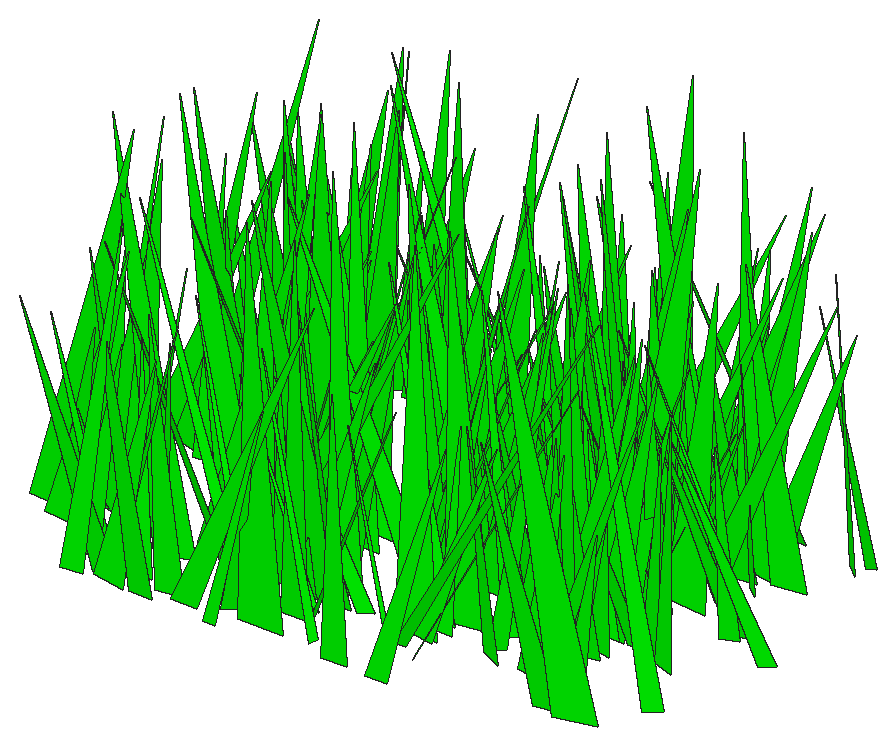
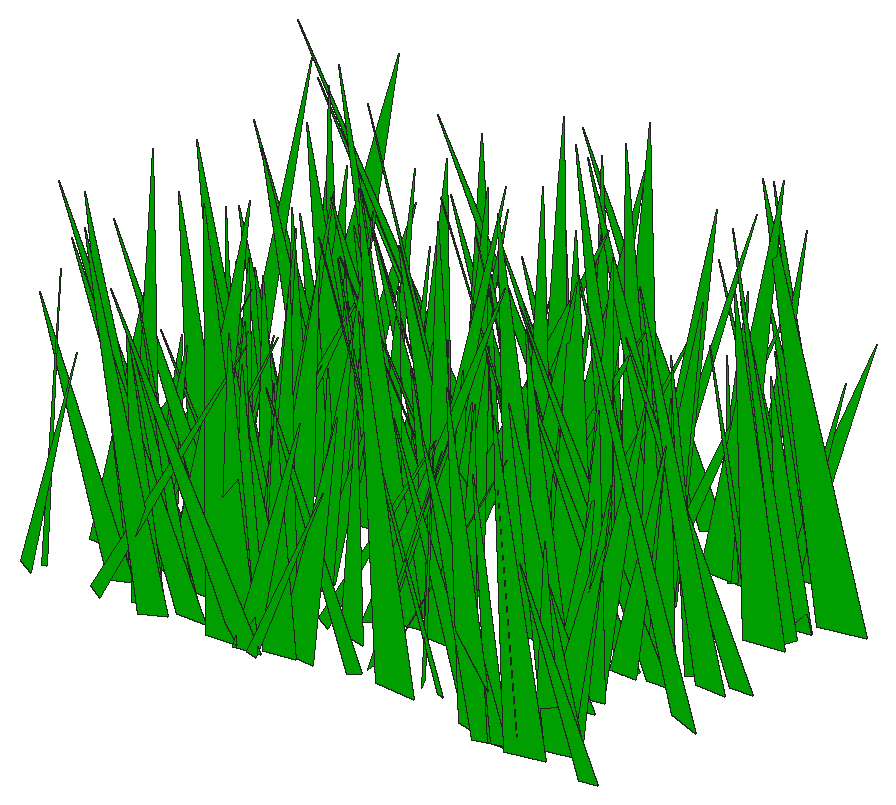
# SketchUp Ruby script. Lengths in inches.
U = 1.inch
M = Sketchup.active_model
def pt(a) = Geom::Point3d.new(a.map { |v| v * U })
def face(e, loops, mat)
  f = e.add_face(loops[0].map { |a| pt(a) })
  loops[1..].each { |l| e.add_face(l.map { |a| pt(a) }).erase! }
  f.material = f.back_material = mat if mat
  f
end
# faces: each face lists its corners as indices into pts; further lists are holes
def faces(e, pts, list, mat = nil) = list.each { |f| face(e, (f[0].is_a?(Array) ? f : [f]).map { |l| l.map { |i| pts[i] } }, mat) }
# xy, xz, yz: faces in a plane at the given z, y or x. An outline is a flat list of corners, or four numbers for a rectangle; further outlines are holes
def ring(l) = l.size == 4 ? [[l[0], l[1]], [l[2], l[1]], [l[2], l[3]], [l[0], l[3]]] : l.each_slice(2).to_a
def flat(e, list, mat, &to3) = list.each { |f| face(e, (f[0].is_a?(Array) ? f : [f]).map { |l| ring(l).map { |u, v| to3.(u, v) } }, mat) }
def xy(e, z, list, mat = nil) = flat(e, list, mat) { |x, y| [x, y, z] }
def xz(e, y, list, mat = nil) = flat(e, list, mat) { |x, z| [x, y, z] }
def yz(e, x, list, mat = nil) = flat(e, list, mat) { |y, z| [x, y, z] }
def lines(e, pts, list) = list.each { |a, b| e.add_line(pt(pts[a]), pt(pts[b])) }
# prism: a flat outline (further loops are holes) pulled along v
def prism(e, loops, v, mat = nil)
  f = face(e, loops, mat); d = Geom::Vector3d.new(v.map { |x| x * U })
  f.pushpull(f.normal.samedirection?(d) ? d.length : -d.length)
end
def box(e, o, s, mat = nil) = prism(e, [[o, [o[0] + s[0], o[1], o[2]], [o[0] + s[0], o[1] + s[1], o[2]], [o[0], o[1] + s[1], o[2]]]], [0, 0, s[2]], mat)
def at(x, y, z, deg = 0) = Geom::Transformation.translation(pt([x, y, z])) * Geom::Transformation.rotation(ORIGIN, Z_AXIS, deg.degrees)
def axes(o, x, y, z) = Geom::Transformation.new([*x, 0, *y, 0, *z, 0, *pt(o).to_a, 1])
def part(name) = M.definitions.add(name)
# library, detail: a bought-in or finely detailed component or shape, given as its bounding box
def library(name, o, s) = part(name).tap { |d| box(d.entities, o, s) }
def detail(e, o, s) = box(e.add_group.entities, o, s)
def put(e, d, t, mat = nil) = e.add_instance(d, t).tap { |i| i.material = mat if mat }
def group(e, t, mat = nil) = e.add_group.tap { |g| g.transformation = t; g.material = mat if mat }.entities
root = M.entities
M.materials.add("[0065_Lime]").color = [0, 255, 0]
c1 = part("fur_instance\#9")
p = [[0.8125,0,1.79],[0.67,-0.02,1.48],[0,-0.11,0],[0,0.11,0]]
faces(c1.entities,p,[[0,1,2,3]])
put(root,c1,axes([50.91,22.23,1.48],[-0.76695,0.80867,0.33759],[-5.73856,-0.11303,0.44668],[0.6003,-0.04733,4.70135]),"[0065_Lime]")
put(root,c1,axes([49.92,33.26,1.48],[2.52942,0.48808,0.58412],[-3.5394,0.33926,0.64151],[0.23083,-0.14633,3.43573]),"[0065_Lime]")
put(root,c1,axes([50.48,21.11,1.48],[-0.67256,-0.6845,0.19925],[4.74683,-0.09985,-0.89267],[1.12113,0.01212,3.89906]),"[0065_Lime]")
put(root,c1,axes([51.94,31.51,1.48],[-4.54403,0.38433,1.74925],[-3.22618,-0.65155,-0.74814],[1.30275,-0.27296,4.24871]),"[0065_Lime]")
put(root,c1,axes([49.74,21.47,1.48],[3.99395,-1.12369,1.36705],[8.17134,0.54771,-0.70957],[0.04674,0.26599,7.23614]),"[0065_Lime]")
put(root,c1,axes([52.3125,31.72,1.48],[-0.7268,-0.77449,0.53828],[5.51485,-0.09001,0.58705],[-0.63479,0.10476,4.48382]),"[0065_Lime]")
put(root,c1,axes([50.54,22.92,1.48],[7.98989,-0.14628,2.13973],[1.33822,1.17114,-0.62341],[-2.49252,0.15988,6.52429]),"[0065_Lime]")
put(root,c1,axes([51.04,23.54,1.48],[2.25533,-0.90203,2.17945],[6.94499,0.31435,-0.39545],[-0.3929,0.37864,5.52033]),"[0065_Lime]")
put(root,c1,axes([49.92,28.72,1.48],[7.6841,0.72682,1.04641],[-5.11442,1.09474,-0.63071],[-1.50059,-0.00934,7.50804]),"[0065_Lime]")
put(root,c1,axes([52.6875,20.2,1.48],[-4.48222,0.17938,1.02633],[-1.535,-0.63027,-0.74423],[0.93025,-0.17572,3.7171]),"[0065_Lime]")
put(root,c1,axes([50.85,22.25,1.48],[2.00716,0.68192,1.98592],[-5.43179,0.24636,0.79769],[0.08265,-0.36953,4.19657]),"[0065_Lime]")
put(root,c1,axes([50.48,20.87,1.48],[3.32906,-0.72326,1.49084],[5.46334,0.44405,-0.85316],[-0.06147,0.29661,4.91258]),"[0065_Lime]")
put(root,c1,axes([50.57,26.65,1.48],[-4.60892,-0.71981,3.549],[5.71561,-0.81095,-0.60041],[3.55095,0.37104,5.5728]),"[0065_Lime]")
put(root,c1,axes([51.49,26.26,1.48],[5.77813,-0.30698,2.05996],[2.54281,0.86465,-0.40144],[-2.17263,0.19556,5.00866]),"[0065_Lime]")
put(root,c1,axes([49.8125,26.12,1.48],[5.45246,0.6124,0.65614],[-4.43057,0.75796,0.65483],[-0.11992,-0.15925,5.63989]),"[0065_Lime]")
put(root,c1,axes([53.56,19.07,1.48],[-3.18516,-0.61642,0.82975],[4.4943,-0.42359,0.87005],[-0.29317,0.20357,4.32299]),"[0065_Lime]")
put(root,c1,axes([52.24,32.25,1.48],[-2.10277,0.6076,0.36206],[-4.26965,-0.30174,0.56101],[0.81554,-0.0131,3.87059]),"[0065_Lime]")
put(root,c1,axes([53.19,26.32,1.48],[-3.37771,-0.97874,1.73276],[7.26758,-0.4748,0.3867],[0.48409,0.29906,6.28475]),"[0065_Lime]")
put(root,c1,axes([53.32,28.98,1.48],[-3.44233,-0.75988,1.52882],[5.71042,-0.47776,0.55002],[0.40921,0.27472,5.18522]),"[0065_Lime]")
put(root,c1,axes([53.21,27.49,1.48],[-3.45068,0.52695,1.19509],[-3.97947,-0.48797,-0.39258],[0.62075,-0.19903,4.12659]),"[0065_Lime]")
put(root,c1,axes([52.51,26.5625,1.48],[-2.79875,-0.72297,0.6651],[5.04299,-0.4087,-0.84615],[1.30717,0.0288,4.68844]),"[0065_Lime]")
put(root,c1,axes([53.12,29.34,1.48],[-3.22496,0.8525,0.55277],[-6.03576,-0.46145,0.54834],[0.91558,-0.03923,5.56179]),"[0065_Lime]")
put(root,c1,axes([51.48,32.38,1.48],[1.93276,-0.94577,0.96552],[6.81569,0.25388,-0.69382],[0.50636,0.19268,5.6536]),"[0065_Lime]")
put(root,c1,axes([52.375,33.1875,1.48],[-1.67785,0.95461,1.59203],[-6.95575,-0.27347,0.64432],[1.2648,-0.23757,5.65537]),"[0065_Lime]")
put(root,c1,axes([53.34,30.1,1.48],[0.33738,-0.67966,0.71284],[4.87263,0.06252,0.47168],[-0.64838,0.1162,3.91559]),"[0065_Lime]")
put(root,c1,axes([52.05,22.86,1.48],[5.4099,-0.08173,1.18749],[0.45868,0.78549,0.42894],[-1.50305,-0.05446,4.40501]),"[0065_Lime]")
put(root,c1,axes([52.31,19.69,1.48],[-1.28397,0.58808,1.45449],[-4.36145,-0.23358,0.61725],[1.30018,-0.20279,3.50693]),"[0065_Lime]")
put(root,c1,axes([54.54,21.14,1.48],[-6.11177,0.83379,2.4404],[-6.48605,-0.87364,-0.74549],[1.46324,-0.38992,6.88873]),"[0065_Lime]")
put(root,c1,axes([52.62,18.63,1.48],[-6.04866,0.41876,3.20472],[-3.14623,-1.00131,0.45529],[3.80849,-0.16212,5.46587]),"[0065_Lime]")
put(root,c1,axes([52.71,29.97,1.48],[1.05104,0.56648,0.01025],[-3.99325,0.14604,0.46794],[0.55353,-0.02209,3.35635]),"[0065_Lime]")
put(root,c1,axes([53.35,32.34,1.48],[7.25224,0.0929,2.18108],[-0.93336,1.0789,0.51345],[-2.5992,-0.12821,5.90123]),"[0065_Lime]")
put(root,c1,axes([53.41,33.16,1.48],[4.50904,-0.4217,1.00213],[2.93431,0.65657,0.52272],[-1.38352,0.01815,4.37469]),"[0065_Lime]")
put(root,c1,axes([55.33,23.34,1.48],[-5.78731,0.88598,2.08157],[-6.6877,-0.82771,-0.49719],[1.25603,-0.32486,6.94378]),"[0065_Lime]")
put(root,c1,axes([55.17,18.71,1.48],[-5.21317,-0.59207,1.74612],[4.53951,-0.75234,0.41909],[1.32453,0.24817,5.4362]),"[0065_Lime]")
put(root,c1,axes([56.38,21.37,1.48],[-6.25595,-0.43733,0.00178],[3.07458,-0.86853,-0.87844],[0.48295,-0.13573,5.61532]),"[0065_Lime]")
put(root,c1,axes([54.44,19.73,1.48],[-3.81203,0.42571,0.97367],[-2.86432,-0.56136,0.80465],[1.55137,0.00959,3.87813]),"[0065_Lime]")
put(root,c1,axes([54.12,21.14,1.48],[-3.81363,-0.33001,1.35293],[2.07947,-0.58422,-0.89694],[1.98947,-0.02196,3.53096]),"[0065_Lime]")
put(root,c1,axes([52.01,27.33,1.48],[5.88229,0.64403,0.51482],[-4.62387,0.81322,0.86661],[0.16303,-0.17262,6.00343]),"[0065_Lime]")
put(root,c1,axes([54.34,33,1.48],[3.98604,0.93129,0.86549],[-6.54901,0.5777,-0.87367],[-1.47219,-0.04836,6.2299]),"[0065_Lime]")
put(root,c1,axes([53.92,18.77,1.48],[-0.50373,0.66106,1.56053],[-4.9413,-0.12675,0.74384],[1.18158,-0.24823,3.77598]),"[0065_Lime]")
put(root,c1,axes([55.15,26.55,1.48],[5.34275,-0.76963,2.59064],[5.69177,0.84019,0.5974],[-2.78312,0.24082,6.19498]),"[0065_Lime]")
put(root,c1,axes([55.07,26.01,1.48],[5.34106,0.58498,2.14604],[-4.12838,0.82961,-0.77951],[-2.6922,-0.11163,5.45286]),"[0065_Lime]")
put(root,c1,axes([53.03,27.32,1.48],[5.09999,-0.34369,0.51708],[2.52545,0.70055,-0.87733],[-0.09331,0.17544,4.51639]),"[0065_Lime]")
put(root,c1,axes([53.69,33.22,1.48],[2.05029,-0.79208,0.95149],[5.72232,0.26129,-0.86987],[0.63048,0.20433,4.8008]),"[0065_Lime]")
put(root,c1,axes([53.94,18.95,1.48],[5.8276,-0.01282,1.10697],[0.25412,0.83464,-0.56111],[-1.34008,0.1025,4.70751]),"[0065_Lime]")
put(root,c1,axes([54.94,23.94,1.48],[3.34017,-0.6062,0.80133],[4.24397,0.48796,0.66477],[-1.25297,0.03678,4.38788]),"[0065_Lime]")
put(root,c1,axes([55.77,19.33,1.48],[1.91514,0.72289,1.34833],[-5.21429,0.31216,-0.70784],[-1.4229,-0.17097,4.40868]),"[0065_Lime]")
put(root,c1,axes([55.1,28.43,1.48],[-4.04577,0.71883,2.20757],[-5.30293,-0.6468,0.62721],[2.32678,-0.22422,5.26794]),"[0065_Lime]")
put(root,c1,axes([56.6,21.78,1.48],[-5.26683,0.16695,0.91476],[-1.02851,-0.75219,0.68212],[1.27222,0.08306,4.33847]),"[0065_Lime]")
put(root,c1,axes([57.63,20.5,1.48],[-7.65891,0.20083,1.23077],[-1.58972,-1.08775,-0.5978],[1.34345,-0.14224,6.30914]),"[0065_Lime]")
put(root,c1,axes([55.63,26.93,1.48],[2.30621,-1.17208,1.2637],[8.43837,0.34044,0.39154],[-0.88473,0.19177,7.02848]),"[0065_Lime]")
put(root,c1,axes([58.35,23.58,1.48],[-6.59593,-0.38825,0.01295],[2.74091,-0.92013,-0.70452],[0.34923,-0.1114,5.77411]),"[0065_Lime]")
put(root,c1,axes([55.45,26.1,1.48],[4.69111,-0.14454,0.46432],[0.90304,0.65379,0.78305],[-0.7539,-0.11623,3.82717]),"[0065_Lime]")
put(root,c1,axes([55.97,23.83,1.48],[7.70775,-0.56988,2.82496],[4.71907,1.128,-0.8941],[-2.49788,0.37258,7.02785]),"[0065_Lime]")
put(root,c1,axes([55.28,22.11,1.48],[5.63845,0.84969,1.66263],[-6.35096,0.78514,0.80506],[-0.6383,-0.30626,6.67677]),"[0065_Lime]")
put(root,c1,axes([58.41,25.96,1.48],[-5.88191,0.76784,0.55283],[-5.39118,-0.83146,0.74571],[1.12088,0.03014,6.48774]),"[0065_Lime]")
put(root,c1,axes([57.48,31.6,1.48],[-5.09105,0.03087,1.59101],[0.16095,-0.75311,0.83036],[1.96168,0.1419,4.06095]),"[0065_Lime]")
put(root,c1,axes([55.9,31.43,1.48],[-2.54793,-0.51736,2.6255],[4.07058,-0.50797,-0.74045],[2.72116,0.27544,3.56598]),"[0065_Lime]")
put(root,c1,axes([56.37,24.12,1.48],[4.58061,-0.00926,0.72159],[-0.03087,0.65183,0.41006],[-0.88902,-0.07036,3.70368]),"[0065_Lime]")
put(root,c1,axes([57.01,21.91,1.48],[6.20209,-0.7948,1.9629],[5.68914,0.92442,0.64918],[-2.33452,0.14124,6.79684]),"[0065_Lime]")
put(root,c1,axes([57.8,29.26,1.48],[-4.14031,0.52741,0.90506],[-3.6265,-0.60243,0.78695],[1.47445,-0.00073,4.477]),"[0065_Lime]")
put(root,c1,axes([56.71,27.5,1.48],[-1.95788,-1.1204,2.34427],[8.30541,-0.33696,-0.80691],[1.70325,0.35518,6.6294]),"[0065_Lime]")
put(root,c1,axes([59.6875,29.92,1.48],[-5.2036,-0.00492,0.04229],[0.04004,-0.72754,0.4245],[0.04822,0.07338,4.21144]),"[0065_Lime]")
put(root,c1,axes([59.3,31.81,1.48],[-5.38794,0.07964,0.65918],[-0.48862,-0.7628,0.44583],[0.85979,0.0656,4.3842]),"[0065_Lime]")
put(root,c1,axes([57.28,26.14,1.48],[-0.40624,0.73286,0.06143],[-5.14035,-0.05806,0.71727],[0.88502,-0.00081,4.19426]),"[0065_Lime]")
put(root,c1,axes([58.06,21.92,1.48],[1.80336,-0.5781,0.49031],[4.09234,0.26311,0.43625],[-0.73588,0.04649,3.62767]),"[0065_Lime]")
put(root,c1,axes([58.4375,25.09,1.48],[6.37602,-0.5878,3.70449],[5.28721,0.99491,-0.73117],[-3.20702,0.47161,6.15963]),"[0065_Lime]")
put(root,c1,axes([59.76,21.28,1.48],[-4.60824,0.10711,0.11861],[-0.70714,-0.63034,0.89686],[0.31983,0.14968,3.69197]),"[0065_Lime]")
put(root,c1,axes([60.9,29.61,1.48],[-8.28329,0.53307,0.34927],[-3.74279,-1.16227,0.71144],[0.75319,0.08686,7.37651]),"[0065_Lime]")
put(root,c1,axes([55.88,26.51,1.48],[8.55097,0.14836,0.91365],[-0.9669,1.20904,-0.59129],[-1.20062,0.08296,6.9833]),"[0065_Lime]")
put(root,c1,axes([57.76,19.76,1.48],[3.06407,-0.42545,0.0148],[2.94808,0.42005,0.78397],[-0.69005,-0.09458,3.41503]),"[0065_Lime]")
put(root,c1,axes([56.57,23.6,1.48],[4.32778,-0.48331,0.42303],[3.47792,0.59883,-0.61607],[0.07001,0.12873,4.45424]),"[0065_Lime]")
put(root,c1,axes([58.37,29.1,1.48],[2.47547,-0.78117,0.14108],[5.46639,0.34663,0.8518],[-1.02653,-0.03795,4.87617]),"[0065_Lime]")
put(root,c1,axes([59,28.67,1.48],[-0.21259,-0.65138,1.66011],[5.04453,-0.00145,0.4083],[-0.45483,0.28833,3.75248]),"[0065_Lime]")
put(root,c1,axes([59.8125,21.87,1.48],[-3.28505,-1.07391,1.09479],[7.75974,-0.45668,0.39469],[0.07902,0.20073,6.75498]),"[0065_Lime]")
put(root,c1,axes([59.96,30.73,1.48],[-5.13041,-0.13974,0.59563],[0.86113,-0.71994,-0.75205],[0.8852,-0.10952,4.18376]),"[0065_Lime]")
put(root,c1,axes([57.15,25.43,1.48],[7.24308,0.20527,1.19815],[-1.33385,1.03654,-0.61555],[-1.58888,0.06558,5.97864]),"[0065_Lime]")
put(root,c1,axes([58.48,29.38,1.48],[-4.3038,-0.99227,2.59386],[7.43876,-0.67256,-0.45504],[2.16775,0.3379,6.71128]),"[0065_Lime]")
put(root,c1,axes([61.0625,22.04,1.48],[-5.10534,0.3444,0.0571],[-2.44346,-0.71273,-0.50051],[-0.20342,-0.0822,4.57922]),"[0065_Lime]")
put(root,c1,axes([57.8125,18.65,1.48],[4.64303,-0.2059,1.00615],[1.6405,0.66228,-0.46734],[-0.99295,0.13138,3.93265]),"[0065_Lime]")
put(root,c1,axes([59.15,19.43,1.48],[2.27554,1.056,2.48484],[-7.9905,0.36872,-0.40927],[-1.4002,-0.38801,6.37384]),"[0065_Lime]")
put(root,c1,axes([57.85,32.51,1.48],[5.11079,-0.85915,0.48487],[6.01909,0.72212,0.89841],[-1.22841,-0.03617,6.41944]),"[0065_Lime]")
put(root,c1,axes([56.45,23.57,1.48],[5.50945,-0.54712,0.24295],[3.90207,0.7685,-0.55548],[0.15185,0.10254,5.45943]),"[0065_Lime]")
put(root,c1,axes([56.61,31.88,1.48],[8.71962,0.24121,1.23734],[-1.84505,1.23683,0.52355],[-1.36248,-0.13121,7.2098]),"[0065_Lime]")
put(root,c1,axes([56.5,19.12,1.48],[6.95279,-0.5172,0.57692],[3.73519,0.97356,-0.53803],[-0.31391,0.12894,6.3764]),"[0065_Lime]")
put(root,c1,axes([59.53,20.5625,1.48],[-5.4228,-0.61009,3.10819],[5.29351,-0.82009,0.71664],[2.33037,0.44318,5.60495]),"[0065_Lime]")
put(root,c1,axes([60.375,21.56,1.48],[-6.07635,-0.24787,1.67223],[2.00294,-0.88877,0.40102],[1.82379,0.15025,5.13099]),"[0065_Lime]")
put(root,c1,axes([58.36,24.62,1.48],[4.95649,0.62607,1.48512],[-4.7256,0.70313,0.50255],[-0.92374,-0.23772,5.39779]),"[0065_Lime]")
put(root,c1,axes([61.23,27.11,1.48],[-8.40057,0.44177,2.08646],[-3.51831,-1.20588,-0.81684],[2.02114,-0.263,7.25011]),"[0065_Lime]")
put(root,c1,axes([60.09,28.51,1.48],[1.85886,-0.6941,1.46111],[5.0808,0.30586,0.59197],[-1.3461,0.19593,4.25203]),"[0065_Lime]")
put(root,c1,axes([62.44,23.31,1.48],[-6.79029,0.59917,0.52613],[-4.31277,-0.94386,-0.8094],[0.01264,-0.16676,6.4716]),"[0065_Lime]")
put(root,c1,axes([59.99,26.36,1.48],[1.96909,-0.67038,1.06054],[4.79826,0.30674,0.60272],[-1.19873,0.12662,4.15467]),"[0065_Lime]")
put(root,c1,axes([59.88,22.55,1.48],[-6.80464,0.60558,3.36486],[-5.1982,-1.0344,-0.71713],[2.94348,-0.4268,6.51232]),"[0065_Lime]")
put(root,c1,axes([62.07,30.61,1.48],[-4.85776,-0.28479,0.11522],[2.02493,-0.67447,0.62299],[-0.16568,0.10694,4.23592]),"[0065_Lime]")
put(root,c1,axes([60.9375,19.72,1.48],[-5.66075,0.10046,1.32359],[-0.90648,-0.81975,-0.48012],[1.52881,-0.11407,4.61621]),"[0065_Lime]")
put(root,c1,axes([58.84,21.86,1.48],[3.4587,-0.5964,1.15342],[4.4747,0.46327,-0.85105],[-0.04143,0.24755,4.37143]),"[0065_Lime]")
put(root,c1,axes([61.43,32.75,1.48],[-1.41536,0.83396,0.29417],[-5.92566,-0.19353,-0.47914],[-0.49049,-0.06844,4.93974]),"[0065_Lime]")
put(root,c1,axes([57.09,23.12,1.48],[8.72174,-0.31722,0.34383],[2.28463,1.22219,-0.55971],[-0.23541,0.10855,7.30677]),"[0065_Lime]")
put(root,c1,axes([59.85,27.92,1.48],[3.64218,-0.49659,0.27106],[3.44871,0.51092,0.70532],[-0.84078,-0.05551,4.06731]),"[0065_Lime]")
put(root,c1,axes([60.81,30.84,1.48],[2.59226,0.5592,1.36677],[-4.10114,0.40508,-0.40716],[-1.35691,-0.15602,3.84172]),"[0065_Lime]")
put(root,c1,axes([61.43,24.76,1.48],[3.01029,1.00004,2.21166],[-7.3505,0.48925,-0.79331],[-2.00297,-0.29247,6.2352]),"[0065_Lime]")
put(root,c1,axes([60.02,26.55,1.48],[1.25248,0.99895,0.96859],[-7.18462,0.15931,0.64134],[0.58162,-0.18328,5.83655]),"[0065_Lime]")
put(root,c1,axes([60.25,29.25,1.48],[4.15878,-1.028,2.33011],[7.80007,0.59479,-0.41799],[-0.94113,0.38698,6.8323]),"[0065_Lime]")
put(root,c1,axes([59.4375,32.42,1.48],[5.21492,-0.26894,0.60312],[1.99426,0.73121,-0.48317],[-0.48561,0.11474,4.49264]),"[0065_Lime]")
put(root,c1,axes([62.55,33.43,1.48],[-4.04811,0.12855,0.50923],[-1.03784,-0.55653,-0.7511],[0.38949,-0.1469,3.2912]),"[0065_Lime]")
put(root,c1,axes([59.95,20.97,1.48],[5.11216,0.05378,0.53262],[-0.25102,0.71161,-0.81361],[-0.7157,0.13456,4.08979]),"[0065_Lime]")
put(root,c1,axes([59.48,26.12,1.48],[5.32264,0.03999,0.09084],[-0.26852,0.74234,-0.54125],[-0.14619,0.09256,4.30177]),"[0065_Lime]")
put(root,c1,axes([62.95,33.2,1.48],[-4.59392,0.54394,0.12316],[-3.81389,-0.64083,0.71276],[0.67936,0.08063,4.83421]),"[0065_Lime]")
put(root,c1,axes([61.87,32.9375,1.48],[-1.7,0.78188,0.30009],[-5.54245,-0.24288,0.43108],[0.6152,-0.02757,4.71291]),"[0065_Lime]")
put(root,c1,axes([62.63,21.125,1.48],[-4.28903,0.00942,0.99222],[-0.2964,-0.61504,-0.65214],[1.18516,-0.11974,3.42769]),"[0065_Lime]")
put(root,c1,axes([62.17,19.12,1.48],[2.68644,0.66194,1.27421],[-4.76929,0.4136,-0.54679],[-1.37785,-0.14103,4.37703]),"[0065_Lime]")
put(root,c1,axes([59.49,26.37,1.48],[6.58653,0.22009,0.01843],[-1.55996,0.92286,-0.42209],[-0.14203,0.0702,5.49076]),"[0065_Lime]")
put(root,c1,axes([63.31,23,1.48],[-6.67138,0.34025,1.21502],[-2.30181,-0.95998,0.64594],[1.67216,0.03603,5.73672]),"[0065_Lime]")
put(root,c1,axes([62.65,25.67,1.48],[1.74422,0.58913,1.28408],[-4.28506,0.28883,-0.5893],[-1.30678,-0.16079,3.6463]),"[0065_Lime]")
put(root,c1,axes([60.8,25.97,1.48],[3.5376,0.81471,1.14572],[-5.96652,0.48257,0.69071],[0.01241,-0.2311,5.48129]),"[0065_Lime]")
put(root,c1,axes([62.66,31.93,1.48],[3.59482,0.87628,2.26092],[-6.55064,0.5671,-0.4738],[-1.92456,-0.29345,5.83578]),"[0065_Lime]")
put(root,c1,axes([62.52,24.32,1.48],[-3.75494,-0.14351,1.46616],[1.35401,-0.56683,0.43523],[1.568,0.1458,3.13521]),"[0065_Lime]")
put(root,c1,axes([63.71,28.56,1.48],[-1.68774,0.54477,0.20803],[-3.86985,-0.23221,-0.39667],[-0.34654,-0.06013,3.41644]),"[0065_Lime]")
put(root,c1,axes([63.01,21.96,1.48],[-4.36766,0.94017,1.57884],[-6.74056,-0.65165,0.6654],[1.76036,-0.16253,6.46516]),"[0065_Lime]")
put(root,c1,axes([63.55,29.07,1.48],[-1.61722,-0.71642,1.69767],[5.50904,-0.2096,0.50838],[-0.01277,0.30614,4.32094]),"[0065_Lime]")
put(root,c1,axes([63.03,26.39,1.48],[2.93343,-0.66512,1.41979],[4.82581,0.45265,0.50863],[-1.47067,0.15866,4.50094]),"[0065_Lime]")
put(root,c1,axes([62.29,27.35,1.48],[5.61244,0.45535,1.2947],[-3.20547,0.8187,-0.45477],[-1.66115,-0.04136,5.25189]),"[0065_Lime]")
put(root,c1,axes([62.32,23.88,1.48],[4.40181,0.56361,0.44438],[-3.8891,0.62028,-0.87293],[-1.12306,0.06107,4.7647]),"[0065_Lime]")
put(root,c1,axes([61.28,24.42,1.48],[8.5414,0.35739,1.32728],[-2.45114,1.22147,-0.58458],[-1.76729,0.03317,7.22556]),"[0065_Lime]")
put(root,c1,axes([64.07,29.79,1.48],[-1.26524,1.09856,0.56818],[-7.83889,-0.17178,-0.42006],[-0.4004,-0.10832,6.42826]),"[0065_Lime]")
put(root,c1,axes([63.96,23.25,1.48],[1.09585,1.16054,0.76639],[-8.22314,0.17089,-0.8917],[-1.2165,-0.10971,6.71799]),"[0065_Lime]")
put(root,c1,axes([63.41,32.97,1.48],[-2.86961,0.8844,0.86003],[-6.25875,-0.42184,0.71871],[1.24832,-0.08197,5.58042]),"[0065_Lime]")
put(root,c1,axes([64.51,27.37,1.48],[-6.95608,0.46861,1.61352],[-3.29199,-1.0156,0.4936],[2.05403,-0.04073,6.25536]),"[0065_Lime]")
put(root,c1,axes([61.64,25.93,1.48],[4.8178,-0.75382,0.66311],[5.42489,0.66577,-0.71704],[0.11942,0.16788,5.82106]),"[0065_Lime]")
put(root,c1,axes([61.6875,24.17,1.48],[6.81668,0.10643,0.68104],[-0.86379,0.95527,0.71826],[-0.72699,-0.13712,5.53247]),"[0065_Lime]")
put(root,c1,axes([63.67,22.5,1.48],[3.76883,-0.22608,1.51495],[1.99768,0.56058,-0.48494],[-1.43757,0.18629,3.29781]),"[0065_Lime]")
put(root,c1,axes([63.4,33.27,1.48],[-0.07333,-1.17159,2.99786],[9.09355,-0.04565,-0.45066],[0.63806,0.51597,6.76723]),"[0065_Lime]")
put(root,c1,axes([64.21,31.43,1.48],[-2.95995,0.63702,0.93245],[-4.48098,-0.4409,0.68192],[1.33668,-0.06742,4.35084]),"[0065_Lime]")
put(root,c1,axes([64.9,25.33,1.48],[-2.83354,-0.54677,0.03454],[3.84202,-0.39426,-0.5967],[0.61774,-0.05591,3.86963]),"[0065_Lime]")
put(root,c1,axes([63.29,25.31,1.48],[1.41923,-0.86794,0.78252],[6.22367,0.18318,-0.66017],[0.5864,0.15649,5.11273]),"[0065_Lime]")
put(root,c1,axes([65.08,29.56,1.48],[-6.34677,-0.48219,2.34206],[3.9047,-0.93938,0.52044],[2.19518,0.27682,5.84567]),"[0065_Lime]")
put(root,c1,axes([64.35,27.5,1.48],[-1.58107,-0.51927,0.54713],[3.65098,-0.23655,-0.54228],[0.88238,0.04833,3.22415]),"[0065_Lime]")
put(root,c1,axes([63.28,21.88,1.48],[3.68808,-0.43184,0.69766],[3.19011,0.50245,-0.73635],[-0.0584,0.17504,3.83488]),"[0065_Lime]")
put(root,c1,axes([64.7,29.76,1.48],[-2.27331,-0.49968,0.73127],[3.48643,-0.34054,-0.62629],[1.13939,0.04507,3.37544]),"[0065_Lime]")
put(root,c1,axes([65.31,23.58,1.48],[-6.50764,0.23238,2.15022],[-1.989,-0.97139,-0.46503],[2.40139,-0.17483,5.44181]),"[0065_Lime]")
put(root,c1,axes([63.59,31.29,1.48],[3.49363,-0.87334,1.4361],[6.45765,0.48114,-0.58956],[-0.20973,0.26656,5.7694]),"[0065_Lime]")
put(root,c1,axes([63.8125,19.08,1.48],[3.77329,0.60173,0.0931],[-4.25611,0.52904,-0.44486],[-0.48574,0.03881,4.62115]),"[0065_Lime]")
put(root,c1,axes([66.24,27.68,1.48],[-6.71563,-0.51563,1.93757],[3.98519,-0.97401,0.4534],[1.80485,0.23206,6.20833]),"[0065_Lime]")
put(root,c1,axes([66.4,31.51,1.48],[-5.00191,0.94983,2.30757],[-7.26659,-0.7061,-0.68249],[0.96725,-0.39286,6.80579]),"[0065_Lime]")
put(root,c1,axes([62.79,33.32,1.48],[5.04034,0.73027,0.34917],[-5.19555,0.69608,0.83939],[0.44627,-0.14399,5.82876]),"[0065_Lime]")
put(root,c1,axes([65.68,22.19,1.48],[-4.06257,-0.41579,0.87649],[2.75991,-0.58913,-0.9009],[1.51648,-0.04171,3.98768]),"[0065_Lime]")
put(root,c1,axes([65.82,30.02,1.48],[1.61771,0.84219,0.39554],[-5.89612,0.23605,-0.88691],[-1.18066,-0.0249,4.97113]),"[0065_Lime]")
put(root,c1,axes([68.53,33.36,1.48],[-6.69317,-0.32485,0.0844],[2.30976,-0.93503,0.59796],[-0.14248,0.10238,5.7288]),"[0065_Lime]")
put(root,c1,axes([65.88,28.3125,1.48],[-3.30615,0.63671,1.63229],[-4.69115,-0.51137,0.39728],[1.59735,-0.18396,4.54519]),"[0065_Lime]")
put(root,c1,axes([65.52,30.15,1.48],[-2.18186,-0.62669,2.27412],[4.95586,-0.38788,-0.43573],[1.77367,0.31287,4.01497]),"[0065_Lime]")
put(root,c1,axes([64.86,29.31,1.48],[4.90307,-0.13042,0.40882],[0.84054,0.68544,0.6574],[-0.6384,-0.09919,4.00546]),"[0065_Lime]")
put(root,c1,axes([65.45,24.89,1.48],[-0.66408,1.0499,2.38572],[-7.92899,-0.15013,0.75356],[1.24849,-0.395,6.05477]),"[0065_Lime]")
put(root,c1,axes([68.2,27.33,1.48],[-4.43988,-0.04005,0.05492],[0.29179,-0.61732,0.52282],[0.0255,0.09074,3.58092]),"[0065_Lime]")
put(root,c1,axes([67.32,30.55,1.48],[0.27881,0.75467,0.28212],[-5.2801,0.0478,-0.83228],[-1.04159,-0.04031,4.29455]),"[0065_Lime]")
put(root,c1,axes([65.76,32.39,1.48],[5.11693,0.49738,1.09889],[-3.50911,0.74246,-0.44955],[-1.42839,-0.04221,5.04097]),"[0065_Lime]")
put(root,c1,axes([65.76,29.11,1.48],[0.71535,1.24088,1.45899],[-8.98166,0.07777,0.69735],[0.72771,-0.25996,7.17278]),"[0065_Lime]")
put(root,c1,axes([66.33,26.87,1.48],[2.98108,0.76058,0.11168],[-5.33579,0.41642,-0.79292],[-0.91948,0.04941,4.96341]),"[0065_Lime]")
put(root,c1,axes([65.5,22.71,1.48],[7.85403,-0.34323,1.66956],[2.35093,1.14068,0.54054],[-2.15693,-0.00653,6.66853]),"[0065_Lime]")
put(root,c1,axes([68.63,25.41,1.48],[-4.20305,-0.47464,0.26566],[3.38898,-0.58326,0.55635],[-0.17673,0.10357,4.35062]),"[0065_Lime]")
put(root,c1,axes([63.03,21.18,1.48],[9.1483,-0.16039,0.06237],[1.14358,1.27969,-0.70668],[0.03182,0.12247,7.46567]),"[0065_Lime]")
put(root,c1,axes([67.19,24.74,1.48],[-3.66366,-0.68484,2.62992],[5.70926,-0.53512,0.59291],[1.26932,0.43022,4.92396]),"[0065_Lime]")
put(root,c1,axes([68.67,29.2,1.48],[-5.29492,0.05278,0.37679],[-0.44574,-0.73662,-0.68657],[0.39622,-0.12331,4.26285]),"[0065_Lime]")
put(root,c1,axes([63.82,20.91,1.48],[7.81531,0.0217,0.01392],[-0.15535,1.09249,0.64675],[-0.00131,-0.11175,6.32533]),"[0065_Lime]")
put(root,c1,axes([67.96,27.79,1.48],[-4.29435,-0.16706,0.95642],[1.40599,-0.60724,0.6226],[0.90513,0.15063,3.57061]),"[0065_Lime]")
put(root,c1,axes([66.8,32.99,1.48],[-2.66176,0.75703,1.0321],[-5.3386,-0.40337,0.80468],[1.46085,-0.09474,4.82122]),"[0065_Lime]")
put(root,c1,axes([67.58,25.38,1.48],[-2.65883,0.48311,0.26242],[-3.40085,-0.37626,0.41318],[0.59894,0.00817,3.51106]),"[0065_Lime]")
put(root,c1,axes([66.22,31.87,1.48],[4.2069,-0.39087,1.03058],[2.98527,0.59046,-0.55868],[-0.65641,0.18029,4.06411]),"[0065_Lime]")
put(root,c1,axes([67.6,23.96,1.48],[1.5068,-0.97559,0.31201],[6.88747,0.21698,0.72699],[-0.95539,0.02558,5.73295]),"[0065_Lime]")
put(root,c1,axes([65.29,32.85,1.48],[5.32152,0.76947,0.6382],[-5.53171,0.74132,0.56801],[-0.04109,-0.14748,6.18498]),"[0065_Lime]")
put(root,c1,axes([66.31,33.39,1.48],[6.25722,-0.57443,1.72526],[4.38996,0.89594,-0.53853],[-1.39227,0.24333,6.05575]),"[0065_Lime]")
put(root,c1,axes([66.86,27.125,1.48],[-1.5402,0.57067,1.14612],[-4.00749,-0.26671,0.88663],[1.55512,-0.1221,3.41993]),"[0065_Lime]")
put(root,c1,axes([68.85,20.85,1.48],[-2.03625,-0.68153,0.93438],[4.97136,-0.26515,0.68755],[-0.35883,0.19396,4.22313]),"[0065_Lime]")
put(root,c1,axes([65.39,30.64,1.48],[6.28756,-0.49303,0.52209],[3.56102,0.87816,-0.58627],[-0.20506,0.13252,5.8274]),"[0065_Lime]")
put(root,c1,axes([67.76,23,1.48],[-5.70386,-0.62209,3.10418],[5.23646,-0.87675,0.47864],[2.59661,0.40158,5.85358]),"[0065_Lime]")
put(root,c1,axes([67.28,22.12,1.48],[-0.94163,0.66624,0.91372],[-4.77241,-0.15854,0.61949],[0.98299,-0.13149,3.88289]),"[0065_Lime]")
put(root,c1,axes([67.79,27.43,1.48],[3.22449,-0.64971,0.89097],[4.52243,0.4767,0.81929],[-1.4581,0.04174,4.51143]),"[0065_Lime]")
put(root,c1,axes([67.57,22.79,1.48],[-1.75565,-0.73704,0.44956],[5.15838,-0.25701,-0.79093],[1.09936,0.02892,4.42909]),"[0065_Lime]")
put(root,c1,axes([67.95,31.75,1.48],[-7.13858,0.54985,3.33434],[-4.70685,-1.09121,-0.63757],[3.15605,-0.38372,6.59099]),"[0065_Lime]")
put(root,c1,axes([68.54,30.56,1.48],[-0.21404,-0.64983,0.81772],[4.70732,-0.01466,0.42484],[-0.48771,0.14368,3.74163]),"[0065_Lime]")
put(root,c1,axes([67.78,24.53,1.48],[-2.76338,-0.65786,1.61804],[4.85114,-0.43652,-0.46552],[1.53032,0.19585,4.3975]),"[0065_Lime]")
put(root,c1,axes([66.82,24.43,1.48],[4.43618,-0.70578,1.26133],[5.22983,0.62136,-0.51952],[-0.53049,0.22355,5.42612]),"[0065_Lime]")
put(root,c1,axes([66.91,28.29,1.48],[4.29662,0.02103,0.21447],[-0.0934,0.5926,-0.70866],[-0.28842,0.12131,3.42449]),"[0065_Lime]")
put(root,c1,axes([67.46,25.5,1.48],[1.50545,0.74732,1.79496],[-5.74538,0.17378,0.76375],[0.38049,-0.33271,4.43063]),"[0065_Lime]")
put(root,c1,axes([69.97,20.8,1.48],[-4.36208,0.99423,1.72364],[-7.38152,-0.59885,-0.78496],[0.25679,-0.32519,6.71541]),"[0065_Lime]")
put(root,c1,axes([67.4,29.21,1.48],[4.01581,-0.2905,0.05322],[2.03293,0.55804,0.57577],[-0.38148,-0.08429,3.62856]),"[0065_Lime]")
put(root,c1,axes([68.15,28.25,1.48],[0.22353,-0.84892,3.02287],[7.07523,-0.01012,-0.44143],[0.49974,0.52305,4.89762]),"[0065_Lime]")
put(root,c1,axes([70.89,28.11,1.48],[-5.70137,0.00991,0.2813],[-0.10145,-0.79932,-0.41668],[0.33806,-0.07271,4.61917]),"[0065_Lime]")
put(root,c1,axes([70.49,27.82,1.48],[-2.51102,-0.53514,0.2124],[3.76954,-0.34069,0.72257],[-0.60185,0.09887,3.63947]),"[0065_Lime]")
put(root,c1,axes([69.95,30.97,1.48],[-2.7179,0.80807,1.31597],[-5.97006,-0.37634,-0.41442],[0.21379,-0.23644,5.15715]),"[0065_Lime]")
put(root,c1,axes([69.2,30.18,1.48],[-4.31723,-0.2358,1.34321],[1.48348,-0.6488,-0.66183],[1.82816,-0.03038,3.70906]),"[0065_Lime]")
put(root,c1,axes([67.34,22.91,1.48],[6.44659,-0.36811,0.30813],[2.54413,0.90039,0.82706],[-0.73052,-0.11274,5.59942]),"[0065_Lime]")
put(root,c1,axes([68.35,31.11,1.48],[2.76339,0.98468,1.40609],[-7.21712,0.37993,0.46903],[-0.08193,-0.2558,6.10923]),"[0065_Lime]")
put(root,c1,axes([69.1,25.45,1.48],[-2.82927,-0.46513,1.22527],[3.25538,-0.44346,-0.66745],[1.6212,0.07875,3.47854]),"[0065_Lime]")
put(root,c1,axes([68.32,32.375,1.48],[3.9638,-0.5566,0.69192],[4.05133,0.54521,-0.65942],[-0.01577,0.1651,4.51019]),"[0065_Lime]")
put(root,c1,axes([70.48,27.49,1.48],[1.41026,0.54456,0.2603],[-3.71614,0.20282,-0.8972],[-1.14506,0.01244,3.2323]),"[0065_Lime]")
put(root,c1,axes([71.08,33.46,1.48],[-4.59539,-0.27305,1.24323],[2.29359,-0.64005,0.8989],[0.92264,0.23115,3.95758]),"[0065_Lime]")
put(root,c1,axes([71.41,22.69,1.48],[-7.68151,0.36544,1.9178],[-2.83844,-1.1156,-0.39889],[2.06534,-0.17402,6.58456]),"[0065_Lime]")
put(root,c1,axes([69.62,20.99,1.48],[0.48235,-0.55598,1.00319],[4.12315,0.04671,-0.44414],[0.41952,0.18013,3.21167]),"[0065_Lime]")
put(root,c1,axes([67.79,30.1,1.48],[6.41006,-0.49385,0.51146],[3.56511,0.89516,-0.59948],[-0.19291,0.1334,5.91601]),"[0065_Lime]")
put(root,c1,axes([70.03,24.9,1.48],[-3.82929,-0.45152,1.6955],[3.27849,-0.60054,-0.45981],[1.9802,0.12114,4.04003]),"[0065_Lime]")
put(root,c1,axes([72.36,26.93,1.48],[-3.18049,0.42731,0.08808],[-2.97301,-0.43168,-0.85251],[-0.6485,-0.11669,3.4763]),"[0065_Lime]")
put(root,c1,axes([70.7,33.03,1.48],[-5.71287,-0.26406,1.77457],[1.59656,-0.85732,-0.87401],[2.3962,-0.05832,4.81316]),"[0065_Lime]")
